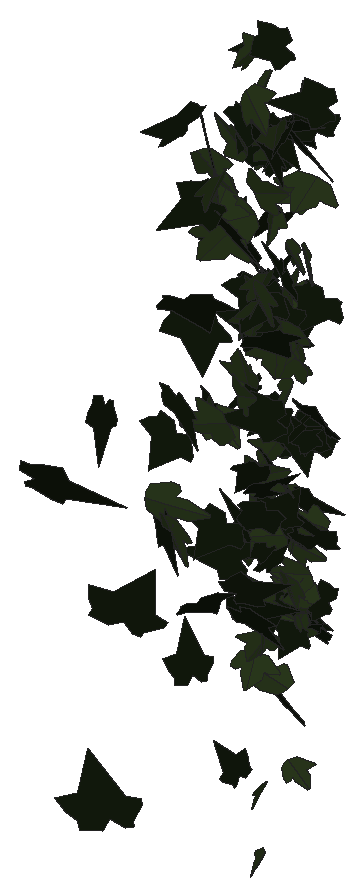
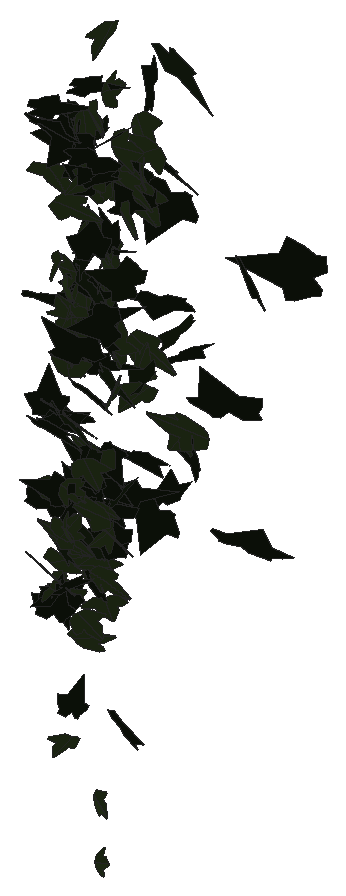
# SketchUp Ruby script. Lengths in inches.
U = 1.inch
M = Sketchup.active_model
def pt(a) = Geom::Point3d.new(a.map { |v| v * U })
def face(e, loops, mat)
  f = e.add_face(loops[0].map { |a| pt(a) })
  loops[1..].each { |l| e.add_face(l.map { |a| pt(a) }).erase! }
  f.material = f.back_material = mat if mat
  f
end
# faces: each face lists its corners as indices into pts; further lists are holes
def faces(e, pts, list, mat = nil) = list.each { |f| face(e, (f[0].is_a?(Array) ? f : [f]).map { |l| l.map { |i| pts[i] } }, mat) }
# xy, xz, yz: faces in a plane at the given z, y or x. An outline is a flat list of corners, or four numbers for a rectangle; further outlines are holes
def ring(l) = l.size == 4 ? [[l[0], l[1]], [l[2], l[1]], [l[2], l[3]], [l[0], l[3]]] : l.each_slice(2).to_a
def flat(e, list, mat, &to3) = list.each { |f| face(e, (f[0].is_a?(Array) ? f : [f]).map { |l| ring(l).map { |u, v| to3.(u, v) } }, mat) }
def xy(e, z, list, mat = nil) = flat(e, list, mat) { |x, y| [x, y, z] }
def xz(e, y, list, mat = nil) = flat(e, list, mat) { |x, z| [x, y, z] }
def yz(e, x, list, mat = nil) = flat(e, list, mat) { |y, z| [x, y, z] }
def lines(e, pts, list) = list.each { |a, b| e.add_line(pt(pts[a]), pt(pts[b])) }
# prism: a flat outline (further loops are holes) pulled along v
def prism(e, loops, v, mat = nil)
  f = face(e, loops, mat); d = Geom::Vector3d.new(v.map { |x| x * U })
  f.pushpull(f.normal.samedirection?(d) ? d.length : -d.length)
end
def box(e, o, s, mat = nil) = prism(e, [[o, [o[0] + s[0], o[1], o[2]], [o[0] + s[0], o[1] + s[1], o[2]], [o[0], o[1] + s[1], o[2]]]], [0, 0, s[2]], mat)
def at(x, y, z, deg = 0) = Geom::Transformation.translation(pt([x, y, z])) * Geom::Transformation.rotation(ORIGIN, Z_AXIS, deg.degrees)
def axes(o, x, y, z) = Geom::Transformation.new([*x, 0, *y, 0, *z, 0, *pt(o).to_a, 1])
def part(name) = M.definitions.add(name)
# library, detail: a bought-in or finely detailed component or shape, given as its bounding box
def library(name, o, s) = part(name).tap { |d| box(d.entities, o, s) }
def detail(e, o, s) = box(e.add_group.entities, o, s)
def put(e, d, t, mat = nil) = e.add_instance(d, t).tap { |i| i.material = mat if mat }
def group(e, t, mat = nil) = e.add_group.tap { |g| g.transformation = t; g.material = mat if mat }.entities
root = M.entities
M.materials.add("1026 AP 7946 SUNNY SIDE UP").color = [254, 231, 186]
M.materials.add("efeu1").color = [18, 25, 13]
M.materials.add("efeu2").color = [43, 57, 29]
c1 = part("ivyleaf_9")
p = [[1.54,2.16,1.25],[1.36,2.04,1.19],[-0.21,0.99,0.68],[-0.71,1.11,0.82],[-0.85,0.86,0.67],[-0.8,0.17,0.21],
  [-0.9,-0.01,0.1],[-0.67,-0.16,-0.02],[-0.08,-0.08,-0.05],[-0.03,-0.6,-0.4],[0.65,-0.88,-0.66],[0.83,-0.6,-0.49],
  [1.29,-0.42,-0.43],[1.8125,-0.07,-0.26],[1.21,0.44,0.15]]
faces(c1.entities,p,[[0,1,2,3,4,5,6,7,8,9,10,11,12,13,14]],"efeu1")
c2 = part("ivyleaf_10")
p = [[0,0.5,-0.03],[-0.0625,2.02,-0.43],[-0.19,2.01,-0.46],[-0.54,1.05,-0.29],[-0.52,0.625,-0.18],[-0.83,0.76,-0.28],
  [-1.16,0.64,-0.33],[-1.15,0.33,-0.24],[-0.77,-0.39,0.02],[-0.3,-0.51,0.16],[0.04,-0.48,0.23],[-0.02,2.01,-0.4375],
  [-0.06,2.01,-0.43],[0.04,-0.49,0.23],[0.67,-0.49,0.14],[1.38,0.36,-0.2],[1.375,0.51,-0.24],[0.81,0.65,-0.19],
  [0.62,0.59,-0.15],[0.6,1.09,-0.28],[0.5,1.23,-0.31]]
faces(c2.entities,p,[[0,1,2,3,4,5,6,7,8,9,10],[11,12,0,13,14,15,16,17,18,19,20]],"efeu2")
put(root,c1,axes([98.35,205.36,260.59],[0.41737,-0.0465,0.31265],[0.49148,-0.04328,-0.26837],[0.10712,0.37976,0.01314]),"1026 AP 7946 SUNNY SIDE UP")
put(root,c1,axes([99.96,205.41,253.97],[-0.63376,-0.03205,0.05036],[0.0748,0.03916,0.39996],[-0.06209,0.3743,-0.03221]),"1026 AP 7946 SUNNY SIDE UP")
put(root,c1,axes([99.56,206.39,257.6],[-0.40496,0.00561,0.28546],[0.45034,-0.03076,0.25443],[0.04525,0.3564,0.02248]),"1026 AP 7946 SUNNY SIDE UP")
put(root,c1,axes([98.47,207.15,261.37],[-0.31224,0.03113,-0.30747],[0.46399,-0.09293,-0.19921],[-0.16085,-0.32851,0.02222]),"1026 AP 7946 SUNNY SIDE UP")
put(root,c1,axes([100.05,207.8,256.01],[-0.24433,-0.20474,0.21585],[0.24467,0.14706,0.26855],[-0.42567,0.20205,0.03047]),"1026 AP 7946 SUNNY SIDE UP")
put(root,c1,axes([99.4,208.44,263.42],[0.4228,0.23776,-0.04129],[-0.02139,-0.04699,-0.36831],[-0.4092,0.24812,-0.02341]),"1026 AP 7946 SUNNY SIDE UP")
put(root,c2,axes([98.875,208.63,258.38],[-0.39103,0.19383,-0.13654],[0.13508,-0.10658,-0.32241],[-0.37252,-0.24212,0.02642]),"1026 AP 7946 SUNNY SIDE UP")
put(root,c1,axes([98.79,208.85,260.2],[-0.22821,-0.24115,0.13548],[-0.08976,-0.11889,-0.29702],[0.45605,-0.14407,0.00933]),"1026 AP 7946 SUNNY SIDE UP")
put(root,c1,axes([98.45,208.91,258.22],[-0.07673,-0.01463,-0.35673],[0.54384,-0.09476,-0.04342],[-0.15635,-0.32244,0.02404]),"1026 AP 7946 SUNNY SIDE UP")
put(root,c1,axes([98.66,209.0625,260.8],[0.14082,-0.28209,0.07792],[0.03055,-0.0744,-0.3158],[0.49519,0.08481,-0.00268]),"1026 AP 7946 SUNNY SIDE UP")
put(root,c2,axes([98.37,208.92,258.59],[0.03192,-0.04341,-0.35848],[0.56239,-0.0594,0.02738],[-0.1056,-0.32949,0.03747]),"1026 AP 7946 SUNNY SIDE UP")
put(root,c1,axes([99.01,208.87,266.85],[-0.28518,0.32364,0.03676],[-0.07501,0.01084,-0.38852],[-0.54665,-0.17033,0.03414]),"1026 AP 7946 SUNNY SIDE UP")
put(root,c1,axes([98.98,209.48,266.48],[0.12441,-0.09139,-0.37158],[0.53155,-0.15439,0.11255],[-0.29375,-0.31808,0.04629]),"1026 AP 7946 SUNNY SIDE UP")
put(root,c1,axes([99.17,209.1,256.625],[0.21629,0.27499,0.07406],[0.0559,0.05702,-0.32361],[-0.47664,0.13147,-0.00435]),"1026 AP 7946 SUNNY SIDE UP")
put(root,c2,axes([99.46,209.32,260.44],[-0.26059,0.02698,0.29437],[-0.46498,-0.05289,-0.1591],[0.05662,-0.31013,0.04825]),"1026 AP 7946 SUNNY SIDE UP")
put(root,c2,axes([99.29,209.46,265.49],[0.00068,-0.34134,0.02499],[0.01024,-0.02778,-0.36576],[0.58127,0.00089,0.00641]),"1026 AP 7946 SUNNY SIDE UP")
put(root,c1,axes([99.1,209.5,264.95],[-0.55291,0.08397,-0.02608],[0.02703,-0.03969,-0.35877],[-0.14647,-0.32429,0.03226]),"1026 AP 7946 SUNNY SIDE UP")
put(root,c1,axes([99.34,209.64,258.12],[-0.42537,-0.10856,-0.02335],[0.04865,-0.01508,-0.29132],[0.18108,-0.25095,0.02343]),"1026 AP 7946 SUNNY SIDE UP")
put(root,c1,axes([99.18,209.61,264.6],[0.51433,-0.13437,-0.0131],[-0.03726,-0.02373,-0.35366],[0.22574,0.30224,-0.02852]),"1026 AP 7946 SUNNY SIDE UP")
put(root,c2,axes([100.05,209.56,267.4375],[0.02803,0.3255,0.10706],[-0.01375,0.09622,-0.34733],[-0.5758,0.01355,0.01351]),"1026 AP 7946 SUNNY SIDE UP")
put(root,c2,axes([99.13,209.67,260.12],[-0.35278,0.18057,-0.01847],[-0.00661,0.02535,0.29456],[0.30826,0.2072,-0.01482]),"1026 AP 7946 SUNNY SIDE UP")
put(root,c1,axes([99.42,209.91,257.27],[-0.20572,-0.02443,0.27813],[-0.40356,-0.10861,-0.13101],[0.18394,-0.26561,0.02363]),"1026 AP 7946 SUNNY SIDE UP")
put(root,c2,axes([99.22,209.76,264.14],[0.48454,0.07273,-0.14712],[-0.25285,0.03912,-0.30638],[-0.08053,0.31479,0.07677]),"1026 AP 7946 SUNNY SIDE UP")
put(root,c1,axes([98.52,209.875,262.03],[-0.28289,-0.2217,-0.14345],[0.17543,0.08547,-0.29418],[0.40048,-0.19404,0.02754]),"1026 AP 7946 SUNNY SIDE UP")
put(root,c1,axes([99.72,209.73,256.3],[0.45196,0.00896,0.01661],[0.02754,-0.02677,-0.28408],[-0.01248,0.26534,-0.02548]),"1026 AP 7946 SUNNY SIDE UP")
put(root,c1,axes([99.58,209.77,256.68],[0.06062,0.0031,0.28015],[0.44168,0.02755,-0.03798],[-0.04705,0.26263,0.00439]),"1026 AP 7946 SUNNY SIDE UP")
put(root,c2,axes([99.7,210.02,262.69],[0.05735,-0.28865,0.11009],[0.04289,-0.10427,-0.31232],[0.52058,0.04039,0.01361]),"1026 AP 7946 SUNNY SIDE UP")
put(root,c2,axes([98.73,210.1,264.8],[-0.02302,0.05313,0.33197],[0.35902,-0.22731,0.04854],[0.39381,0.21033,-0.02485]),"1026 AP 7946 SUNNY SIDE UP")
put(root,c2,axes([99.875,210.09,255.69],[0.01139,0.00861,0.27351],[0.25993,-0.20464,0.00023],[0.34723,0.15291,-0.00914]),"1026 AP 7946 SUNNY SIDE UP")
put(root,c1,axes([98.68,210.17,260.2],[0.09152,-0.21288,0.16946],[0.05974,-0.15721,-0.23726],[0.4492,0.06428,-0.00297]),"1026 AP 7946 SUNNY SIDE UP")
put(root,c2,axes([98.5625,210.07,265.44],[-0.33815,0.04835,-0.21784],[0.31264,-0.0944,-0.21769],[-0.17041,-0.26913,0.03288]),"1026 AP 7946 SUNNY SIDE UP")
put(root,c2,axes([99.89,210.125,255.66],[-0.22742,-0.18989,0.10883],[-0.07143,-0.09729,-0.24924],[0.36062,-0.13902,0.01926]),"1026 AP 7946 SUNNY SIDE UP")
put(root,c2,axes([99.76,210.0625,263.11],[-0.39639,0.17976,-0.10603],[0.12118,-0.07329,-0.31616],[-0.32871,-0.24379,0.01131]),"1026 AP 7946 SUNNY SIDE UP")
put(root,c2,axes([99.42,210.08,264.55],[0.32811,-0.12751,-0.26503],[-0.39361,0.08954,-0.24358],[0.25721,0.29968,-0.03468]),"1026 AP 7946 SUNNY SIDE UP")
put(root,c1,axes([99.47,209.97,256.19],[0.17952,0.04866,0.27376],[0.42925,0.04339,-0.12049],[-0.10033,0.2727,-0.02566]),"1026 AP 7946 SUNNY SIDE UP")
put(root,c1,axes([99.02,209.99,263.93],[-0.22191,-0.0625,0.26231],[0.36683,0.11738,0.15661],[-0.22547,0.25247,-0.00338]),"1026 AP 7946 SUNNY SIDE UP")
put(root,c2,axes([99.25,210.2,260.56],[-0.20039,0.08895,0.23792],[0.34624,-0.08987,0.15405],[0.20919,0.23395,-0.02706]),"1026 AP 7946 SUNNY SIDE UP")
put(root,c1,axes([99.73,210.33,262.87],[-0.34504,-0.2249,0.04663],[0.05588,-0.08997,-0.31316],[0.38582,-0.1881,0.08705]),"1026 AP 7946 SUNNY SIDE UP")
put(root,c2,axes([98.88,210.08,264.52],[0.47175,-0.0398,-0.0344],[0.06102,0.02967,0.29872],[-0.06099,-0.27812,0.03278]),"1026 AP 7946 SUNNY SIDE UP")
put(root,c2,axes([99.76,210.24,263.23],[-0.04685,-0.30318,0.06597],[0.00186,-0.06593,-0.32675],[0.52655,-0.02674,0.00702]),"1026 AP 7946 SUNNY SIDE UP")
put(root,c1,axes([99.97,210.34,260.25],[-0.29856,-0.04454,0.23246],[-0.33859,-0.09078,-0.19365],[0.16632,-0.26475,0.02305]),"1026 AP 7946 SUNNY SIDE UP")
put(root,c2,axes([98.74,210.1,259.97],[0.19668,0.22479,0.16295],[0.133,0.12744,-0.26876],[-0.43833,0.13953,-0.00843]),"1026 AP 7946 SUNNY SIDE UP")
put(root,c2,axes([99.53,210.27,255.02],[0.3093,0.18333,-0.07376],[-0.06143,-0.06427,-0.27687],[-0.32821,0.1848,-0.01769]),"1026 AP 7946 SUNNY SIDE UP")
put(root,c2,axes([99.29,210.3,260.9375],[-0.42334,0.08472,-0.03266],[-0.03727,0.03323,0.28124],[0.1489,0.24917,-0.02246]),"1026 AP 7946 SUNNY SIDE UP")
put(root,c2,axes([99.48,210.41,262.32],[-0.20555,-0.27651,-0.00342],[0.00842,-0.00262,-0.32315],[0.46932,-0.12106,0.0043]),"1026 AP 7946 SUNNY SIDE UP")
put(root,c1,axes([99.74,210.27,261.95],[0.34058,0.21854,0.04123],[0.06586,0.01268,-0.31672],[-0.37007,0.20338,-0.01842]),"1026 AP 7946 SUNNY SIDE UP")
put(root,c1,axes([99.07,210.37,252.375],[-0.05526,0.10571,0.25192],[-0.17174,0.21144,-0.11441],[-0.4005,-0.10525,0.0143]),"1026 AP 7946 SUNNY SIDE UP")
put(root,c1,axes([99.05,210.69,263.43],[0.01719,-0.04619,0.27499],[0.08735,-0.25227,-0.05414],[0.43536,0.05244,0.00001]),"1026 AP 7946 SUNNY SIDE UP")
put(root,c1,axes([99.11,210.56,257.54],[-0.03022,-0.22204,0.11141],[0.01017,0.10681,0.23995],[-0.41825,0.01864,-0.00222]),"1026 AP 7946 SUNNY SIDE UP")
put(root,c1,axes([99.4375,210.71,257.95],[0.02812,0.04202,-0.25805],[-0.06926,-0.23829,-0.05069],[-0.41046,0.04308,-0.00912]),"1026 AP 7946 SUNNY SIDE UP")
put(root,c1,axes([100.22,210.38,261.875],[-0.12311,0.07376,-0.29072],[-0.32619,0.19324,0.11344],[0.35111,0.20538,0.00346]),"1026 AP 7946 SUNNY SIDE UP")
put(root,c1,axes([99.375,210.85,265.72],[0.09806,-0.25659,0.17105],[0.05602,-0.15977,-0.28379],[0.51308,0.06648,-0.00171]),"1026 AP 7946 SUNNY SIDE UP")
put(root,c1,axes([99.38,210.7,255.46],[-0.05681,0.12459,0.21498],[0.10977,-0.18854,0.13525],[0.38341,0.07243,-0.00687]),"1026 AP 7946 SUNNY SIDE UP")
put(root,c2,axes([99.98,210.72,260.78],[0.2305,-0.24549,0.00272],[-0.01006,-0.00984,-0.30029],[0.41672,0.13555,-0.00876]),"1026 AP 7946 SUNNY SIDE UP")
put(root,c2,axes([98.57,210.83,264.26],[0.22856,-0.22758,0.14244],[0.09258,-0.12551,-0.28438],[0.44044,0.14448,-0.01414]),"1026 AP 7946 SUNNY SIDE UP")
put(root,c2,axes([99.35,210.63,256.02],[0.09033,0.04311,0.24894],[0.34956,0.10757,-0.07048],[-0.19548,0.21229,-0.011]),"1026 AP 7946 SUNNY SIDE UP")
put(root,c2,axes([98.93,210.57,265.6],[-0.14561,0.07022,-0.30218],[-0.3331,0.20454,0.12078],[0.3665,0.21379,-0.01028]),"1026 AP 7946 SUNNY SIDE UP")
put(root,c1,axes([99.15,210.77,260.48],[-0.31264,0.13027,-0.11509],[0.116,-0.09068,-0.24047],[-0.26421,-0.19396,0.03061]),"1026 AP 7946 SUNNY SIDE UP")
put(root,c2,axes([99.7,210.73,261.47],[-0.33834,-0.21409,-0.00647],[0.04213,-0.01869,-0.31166],[0.36102,-0.19846,0.03031]),"1026 AP 7946 SUNNY SIDE UP")
put(root,c2,axes([99.6,210.8125,257.47],[-0.16397,-0.00773,0.23724],[-0.30815,-0.13623,-0.09166],[0.21645,-0.19981,0.04923]),"1026 AP 7946 SUNNY SIDE UP")
put(root,c1,axes([98.87,210.97,265.96],[-0.11599,-0.21867,0.13206],[-0.03282,-0.12583,-0.24637],[0.42734,-0.06902,0.01692]),"1026 AP 7946 SUNNY SIDE UP")
put(root,c1,axes([99.26,210.91,261.71],[-0.10036,0.00958,0.28925],[-0.41586,-0.11857,-0.05457],[0.1936,-0.24973,0.03273]),"1026 AP 7946 SUNNY SIDE UP")
put(root,c2,axes([99.6875,210.81,254.34],[0.16013,0.11563,0.212],[-0.29715,-0.09955,0.15128],[0.24802,-0.19392,0.04437]),"1026 AP 7946 SUNNY SIDE UP")
put(root,c1,axes([99.22,210.81,258.76],[0.09148,0.15258,-0.19059],[-0.07873,-0.1742,-0.17537],[-0.39277,0.07045,-0.00924]),"1026 AP 7946 SUNNY SIDE UP")
put(root,c2,axes([99.22,210.85,264.59],[-0.29118,0.05271,0.26495],[0.41759,-0.03167,0.18984],[0.0956,0.29888,-0.02226]),"1026 AP 7946 SUNNY SIDE UP")
put(root,c1,axes([99.9375,210.98,255.51],[-0.16818,-0.18523,0.07283],[-0.04126,-0.0668,-0.22559],[0.33387,-0.10156,0.00881]),"1026 AP 7946 SUNNY SIDE UP")
put(root,c1,axes([99.82,210.95,266.16],[-0.27914,0.11302,-0.24632],[0.28276,-0.16294,-0.21406],[-0.33371,-0.2326,0.02466]),"1026 AP 7946 SUNNY SIDE UP")
put(root,c2,axes([99.59,210.83,266.08],[-0.08557,-0.30883,-0.05674],[0.03112,0.0466,-0.33416],[0.52989,-0.05261,0.01046]),"1026 AP 7946 SUNNY SIDE UP")
put(root,c1,axes([99.35,210.875,257.21],[-0.39657,0.12982,-0.02901],[0.02262,-0.03506,-0.28545],[-0.22459,-0.23276,0.02248]),"1026 AP 7946 SUNNY SIDE UP")
put(root,c2,axes([100,210.84,261.29],[-0.37376,0.08746,0.16762],[-0.28694,-0.02359,-0.24247],[-0.09655,-0.26848,0.07174]),"1026 AP 7946 SUNNY SIDE UP")
put(root,c2,axes([99.76,210.85,261.9375],[-0.50642,0.03641,-0.00558],[0.00287,-0.03284,-0.32033],[-0.06249,-0.29657,0.03054]),"1026 AP 7946 SUNNY SIDE UP")
put(root,c1,axes([99.61,210.95,260.11],[-0.39967,0.02816,-0.06221],[0.09151,-0.03766,-0.25233],[-0.06135,-0.23965,0.02887]),"1026 AP 7946 SUNNY SIDE UP")
put(root,c1,axes([99.6875,210.81,262.02],[-0.41622,-0.11338,0.14799],[0.19169,0.08689,0.28886],[-0.2378,0.26849,-0.02618]),"1026 AP 7946 SUNNY SIDE UP")
put(root,c1,axes([99.21,211.09,262.22],[-0.05455,0.00128,0.29147],[-0.08157,-0.26985,-0.00849],[0.45488,-0.04824,0.03343]),"1026 AP 7946 SUNNY SIDE UP")
put(root,c2,axes([99.87,210.9,256.53],[-0.32673,0.12551,-0.02444],[0.01533,-0.03076,-0.24543],[-0.21653,-0.19157,0.0195]),"1026 AP 7946 SUNNY SIDE UP")
put(root,c2,axes([99.17,210.93,258.52],[-0.32272,-0.03574,0.20586],[0.32086,0.03781,0.20762],[-0.08828,0.26808,0.00205]),"1026 AP 7946 SUNNY SIDE UP")
put(root,c1,axes([99.18,210.86,258.21],[0.26648,0.2094,-0.01231],[-0.00865,0.02157,0.27989],[0.35618,-0.15614,0.01601]),"1026 AP 7946 SUNNY SIDE UP")
put(root,c2,axes([99.14,210.9375,256],[0.14957,-0.04587,-0.25287],[-0.36761,0.09306,-0.10479],[0.17574,0.23369,-0.004]),"1026 AP 7946 SUNNY SIDE UP")
put(root,c1,axes([99.24,210.83,261.33],[-0.03506,0.07967,0.25524],[-0.15412,0.21959,-0.0843],[-0.39613,-0.09249,0.01021]),"1026 AP 7946 SUNNY SIDE UP")
put(root,c2,axes([99.01,210.81,256.97],[-0.01147,-0.04794,-0.27636],[0.12326,0.24717,-0.04785],[0.42724,-0.0726,0.00638]),"1026 AP 7946 SUNNY SIDE UP")
put(root,c1,axes([99.53,210.96,257.75],[-0.25806,0.07715,0.17843],[0.25066,-0.0751,0.18146],[0.18278,0.21193,0.00307]),"1026 AP 7946 SUNNY SIDE UP")
put(root,c2,axes([100.04,211.05,256.68],[0.1776,-0.02658,-0.23618],[-0.36504,0.04776,-0.11485],[0.09264,0.23912,0.0002]),"1026 AP 7946 SUNNY SIDE UP")
put(root,c1,axes([99.36,210.91,256.7],[-0.18085,0.24062,-0.02334],[-0.01148,0.02428,0.28204],[0.4105,0.10669,-0.00239]),"1026 AP 7946 SUNNY SIDE UP")
put(root,c2,axes([98.65,211.3,267.25],[-0.00314,-0.02068,0.30948],[0.12809,-0.27942,-0.02476],[0.47547,0.07514,0.00871]),"1026 AP 7946 SUNNY SIDE UP")
put(root,c1,axes([98.17,211.17,263.02],[0.2868,-0.17602,0.17296],[0.24521,-0.08582,-0.25935],[0.32637,0.21915,0.04286]),"1026 AP 7946 SUNNY SIDE UP")
put(root,c1,axes([99.69,211.21,265.84],[0.3217,-0.19433,0.13778],[0.12099,-0.11391,-0.29005],[0.35169,0.21694,-0.02624]),"1026 AP 7946 SUNNY SIDE UP")
put(root,c2,axes([99.85,211.11,255.39],[-0.3141,-0.10176,0.04826],[0.05658,0.03546,0.22602],[-0.18122,0.18744,-0.01308]),"1026 AP 7946 SUNNY SIDE UP")
put(root,c2,axes([99.28,211.22,264.03],[0.00014,0.22831,-0.18252],[-0.04685,-0.17265,-0.2457],[-0.48448,0.01676,0.02371]),"1026 AP 7946 SUNNY SIDE UP")
put(root,c2,axes([100.02,211.15,256.11],[0.19882,0.10734,0.19535],[-0.26263,-0.09661,0.1671],[0.2423,-0.1928,0.02083]),"1026 AP 7946 SUNNY SIDE UP")
put(root,c1,axes([99.64,211.21,262.6875],[0.06695,-0.26085,0.11524],[-0.02146,0.1126,0.2729],[-0.44669,-0.04451,0.00416]),"1026 AP 7946 SUNNY SIDE UP")
put(root,c2,axes([100.15,211.21,264.95],[0.4721,0.04968,-0.08729],[-0.13058,-0.03551,-0.30214],[-0.0976,0.28781,-0.01801]),"1026 AP 7946 SUNNY SIDE UP")
put(root,c2,axes([98.7,211.15,260.24],[-0.11051,0.26959,-0.0053],[-0.0047,0.00612,0.28704],[0.42401,0.07033,0.0018]),"1026 AP 7946 SUNNY SIDE UP")
put(root,c2,axes([100.25,211.25,257.71],[0.07094,0.05696,0.24772],[-0.3257,-0.13001,0.06978],[0.23783,-0.19504,0.02167]),"1026 AP 7946 SUNNY SIDE UP")
put(root,c1,axes([99.4,211.16,257.71],[0.05289,-0.16562,-0.17331],[-0.02303,0.15958,-0.17775],[0.38991,0.03189,0.01301]),"1026 AP 7946 SUNNY SIDE UP")
put(root,c1,axes([99.89,211.28,256.625],[-0.23835,0.07544,-0.15211],[0.18311,-0.09748,-0.16974],[-0.20457,-0.17515,0.0253]),"1026 AP 7946 SUNNY SIDE UP")
put(root,c2,axes([99.48,211.37,260.97],[0.01831,0.00663,0.24795],[0.19774,-0.20048,-0.00246],[0.33983,0.1163,-0.01193]),"1026 AP 7946 SUNNY SIDE UP")
put(root,c1,axes([99.04,211.29,258.6875],[0.22908,-0.17962,0.06306],[0.03517,-0.06076,-0.24049],[0.32023,0.13517,-0.0187]),"1026 AP 7946 SUNNY SIDE UP")
put(root,c1,axes([100.22,211.25,257.33],[0.22393,-0.01427,0.21462],[-0.32394,0.06704,0.14035],[-0.10804,-0.23059,0.02402]),"1026 AP 7946 SUNNY SIDE UP")
put(root,c2,axes([99.58,211.06,262.29],[-0.01787,-0.15429,-0.26586],[0.04302,0.24505,-0.16207],[0.49152,-0.02706,0.00452]),"1026 AP 7946 SUNNY SIDE UP")
put(root,c1,axes([99.6875,211.32,259.58],[-0.13011,-0.2571,-0.11429],[0.08681,0.09688,-0.27681],[0.43072,-0.09719,0.02127]),"1026 AP 7946 SUNNY SIDE UP")
put(root,c2,axes([99.98,211.09,255.73],[-0.00107,0.11235,0.20324],[-0.10687,0.18036,-0.11287],[-0.35666,-0.05438,0.03321]),"1026 AP 7946 SUNNY SIDE UP")
put(root,c1,axes([99.99,211.21,255.4375],[0.06892,0.19012,-0.09277],[-0.02844,-0.08756,-0.20935],[-0.35532,0.04389,-0.00124]),"1026 AP 7946 SUNNY SIDE UP")
put(root,c1,axes([100.16,211.26,259.61],[-0.35928,0.12016,0.09299],[-0.15671,0.00823,-0.25753],[-0.19498,-0.22804,0.03564]),"1026 AP 7946 SUNNY SIDE UP")
put(root,c1,axes([99.21,211.11,262.63],[-0.16447,0.22186,-0.06512],[-0.02818,0.06223,0.25985],[0.39082,0.09785,-0.00867]),"1026 AP 7946 SUNNY SIDE UP")
put(root,c1,axes([99.01,211.34,263.57],[0.24593,0.16464,0.19365],[-0.22266,-0.12219,0.23261],[0.34726,-0.19495,0.01201]),"1026 AP 7946 SUNNY SIDE UP")
put(root,c1,axes([100.05,211.22,259.34],[0.07639,0.05727,0.26273],[-0.35616,0.14534,0.00692],[-0.23473,-0.20189,0.07501]),"1026 AP 7946 SUNNY SIDE UP")
put(root,c2,axes([98.91,211.43,266.69],[0.2101,-0.21071,0.13969],[0.08993,-0.12312,-0.26287],[0.41353,0.13383,-0.01381]),"1026 AP 7946 SUNNY SIDE UP")
put(root,c1,axes([99.86,211.29,259.71],[-0.28348,0.19884,-0.03427],[0.02073,-0.03487,-0.27813],[-0.34199,-0.16694,0.01154]),"1026 AP 7946 SUNNY SIDE UP")
put(root,c2,axes([98.79,211.38,257.68],[-0.02752,-0.01495,-0.28732],[0.40801,-0.10402,-0.01164],[-0.16211,-0.25927,0.01947]),"1026 AP 7946 SUNNY SIDE UP")
put(root,c2,axes([99.53,211.47,258.0625],[-0.06823,-0.16206,0.17844],[-0.05274,-0.16604,-0.18092],[0.39369,-0.05033,0.00669]),"1026 AP 7946 SUNNY SIDE UP")
put(root,c1,axes([99.5625,211.55,255.875],[-0.17758,-0.11922,0.19374],[-0.16107,-0.16026,-0.16837],[0.31189,-0.15064,0.02336]),"1026 AP 7946 SUNNY SIDE UP")
put(root,c1,axes([99.54,211.2,265.96],[0.3462,0.19531,0.04182],[0.06913,0.01013,-0.30135],[-0.33012,0.20694,-0.01925]),"1026 AP 7946 SUNNY SIDE UP")
put(root,c1,axes([99.99,211.47,259.76],[0.39393,-0.13354,-0.01157],[0.03222,0.01487,0.28584],[-0.22491,-0.23176,0.02069]),"1026 AP 7946 SUNNY SIDE UP")
put(root,c2,axes([99.52,211.52,257.21],[0.09278,-0.07585,0.20764],[0.17351,-0.16611,-0.10219],[0.30981,0.11575,-0.00495]),"1026 AP 7946 SUNNY SIDE UP")
put(root,c2,axes([98.6875,211.54,249.98],[0.05079,-0.09457,0.19027],[0.09863,-0.1743,-0.10396],[0.3118,0.07054,0.00189]),"1026 AP 7946 SUNNY SIDE UP")
put(root,c1,axes([99.02,211.23,265],[-0.13311,-0.02278,0.29729],[0.40094,0.14818,0.0864],[-0.25187,0.24793,-0.01959]),"1026 AP 7946 SUNNY SIDE UP")
put(root,c2,axes([99.92,211.49,255.69],[0.08556,0.12654,-0.15939],[-0.09709,-0.13924,-0.14776],[-0.31939,0.07623,0.00222]),"1026 AP 7946 SUNNY SIDE UP")
put(root,c2,axes([99.59,211.47,256.96],[0.00259,-0.03096,-0.26117],[0.3572,-0.12531,0.01672],[-0.21471,-0.20885,0.02466]),"1026 AP 7946 SUNNY SIDE UP")
put(root,c1,axes([100.18,211.5625,266.46],[-0.24309,-0.04325,0.25379],[-0.35259,-0.10498,-0.1644],[0.17509,-0.27146,0.02128]),"1026 AP 7946 SUNNY SIDE UP")
put(root,c2,axes([99.63,211.32,252.32],[0.1404,0.17995,0.10558],[0.0706,0.08684,-0.21081],[-0.33917,0.09256,-0.00018]),"1026 AP 7946 SUNNY SIDE UP")
put(root,c1,axes([100.4,211.35,256.07],[-0.26696,0.16634,0.10432],[-0.13673,0.05407,-0.24363],[-0.27313,-0.18965,0.01999]),"1026 AP 7946 SUNNY SIDE UP")
put(root,c2,axes([99.45,211.53,262.52],[0.07548,-0.16307,-0.17241],[0.0874,-0.15053,0.17869],[-0.37653,-0.06763,0.00691]),"1026 AP 7946 SUNNY SIDE UP")
put(root,c1,axes([98.875,211.39,265.71],[-0.11224,-0.12826,-0.25944],[0.231,0.19908,-0.15083],[0.40117,-0.15052,0.01427]),"1026 AP 7946 SUNNY SIDE UP")
put(root,c2,axes([99.59,211.51,257.09],[-0.22589,-0.10684,-0.14306],[-0.17118,-0.0856,0.18147],[-0.23234,0.16694,0.00539]),"1026 AP 7946 SUNNY SIDE UP")
put(root,c1,axes([99.64,211.3,255.6],[0.01717,-0.00122,-0.23107],[0.06875,0.21223,0.00372],[0.35986,-0.04049,0.01032]),"1026 AP 7946 SUNNY SIDE UP")
put(root,c2,axes([99.61,211.49,264.48],[0.19349,0.03113,-0.25926],[-0.40004,-0.05757,-0.12726],[-0.11098,0.26176,0.00672]),"1026 AP 7946 SUNNY SIDE UP")
put(root,c2,axes([99.0625,211.28,265.28],[-0.14348,-0.17335,-0.24462],[0.23211,0.18682,-0.19868],[0.39834,-0.1713,0.02765]),"1026 AP 7946 SUNNY SIDE UP")
put(root,c2,axes([99.5,211.47,260.81],[-0.43357,0.0335,0.10068],[0.15081,-0.01906,0.28595],[0.05961,0.29186,0.00885]),"1026 AP 7946 SUNNY SIDE UP")
put(root,c1,axes([98.44,211.45,262.12],[0.38986,-0.10584,0.11427],[0.1406,-0.07289,-0.27648],[0.19667,0.26191,-0.02886]),"1026 AP 7946 SUNNY SIDE UP")
put(root,c1,axes([99.13,211.625,267.34],[-0.26632,-0.07318,0.22253],[-0.29554,-0.11715,-0.18563],[0.23181,-0.23343,0.019]),"1026 AP 7946 SUNNY SIDE UP")
put(root,c1,axes([100.1,211.61,262.31],[-0.39203,-0.13921,-0.00628],[0.0523,-0.04342,-0.28364],[0.23056,-0.22686,0.05367]),"1026 AP 7946 SUNNY SIDE UP")
put(root,c1,axes([99.81,211.5625,255.23],[0.33997,-0.12251,0.08829],[-0.10002,0.06234,0.25541],[-0.21346,-0.22433,0.02095]),"1026 AP 7946 SUNNY SIDE UP")
put(root,c1,axes([100.08,211.6,259.43],[-0.44113,0.00021,0.00458],[-0.00726,-0.02861,-0.27691],[0.00044,-0.25832,0.02703]),"1026 AP 7946 SUNNY SIDE UP")
put(root,c2,axes([99.35,211.61,263.12],[-0.111,0.0792,-0.2216],[0.1941,-0.17407,-0.11186],[-0.3242,-0.13133,0.0089]),"1026 AP 7946 SUNNY SIDE UP")
put(root,c1,axes([99.59,211.5,257.95],[0.20621,-0.022,0.18889],[0.27849,-0.0694,-0.13095],[0.1176,0.2029,-0.02111]),"1026 AP 7946 SUNNY SIDE UP")
put(root,c2,axes([98.99,211.56,258.82],[-0.28732,-0.1289,0.09156],[-0.08916,-0.07396,-0.22722],[0.24868,-0.17545,0.02432]),"1026 AP 7946 SUNNY SIDE UP")
put(root,c2,axes([98.67,211.6,251.42],[0.07658,-0.19462,0.07547],[0.0192,-0.07357,-0.20703],[0.32703,0.04989,-0.00551]),"1026 AP 7946 SUNNY SIDE UP")
put(root,c2,axes([99.02,211.63,255.4],[-0.1744,-0.16559,0.1459],[-0.10483,-0.12661,-0.20567],[0.32719,-0.12883,0.01187]),"1026 AP 7946 SUNNY SIDE UP")
put(root,c2,axes([99.43,211.45,262.05],[0.32505,0.07629,-0.1171],[0.15524,0.06655,0.22001],[0.16667,-0.21076,0.02346]),"1026 AP 7946 SUNNY SIDE UP")
put(root,c1,axes([100.09,211.43,266],[-0.45772,0.03366,-0.02371],[-0.03209,0.02496,0.30114],[0.05571,0.29095,-0.02136]),"1026 AP 7946 SUNNY SIDE UP")
put(root,c2,axes([99.71,211.59,263.16],[-0.16351,0.22964,-0.07755],[0.03369,-0.07341,-0.26743],[-0.40893,-0.09787,0.00898]),"1026 AP 7946 SUNNY SIDE UP")
put(root,c1,axes([99.27,211.67,253.26],[0.26909,-0.1748,0.03752],[-0.02126,0.03899,0.2516],[-0.28028,-0.17078,0.01694]),"1026 AP 7946 SUNNY SIDE UP")
put(root,c1,axes([99.15,211.54,261.25],[-0.1484,-0.00739,0.28582],[0.42858,-0.05794,0.09358],[0.08261,0.28731,0.02797]),"1026 AP 7946 SUNNY SIDE UP")
put(root,c1,axes([98.66,211.76,265.46],[-0.19126,-0.14187,0.14574],[-0.12852,-0.1158,-0.19526],[0.31039,-0.13537,0.00895]),"1026 AP 7946 SUNNY SIDE UP")
